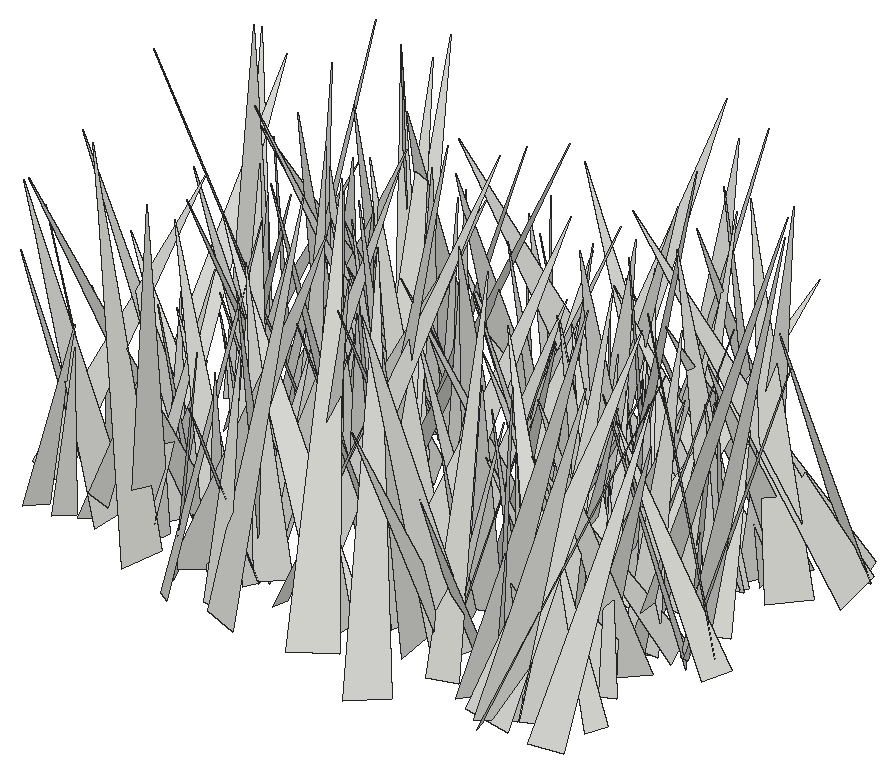
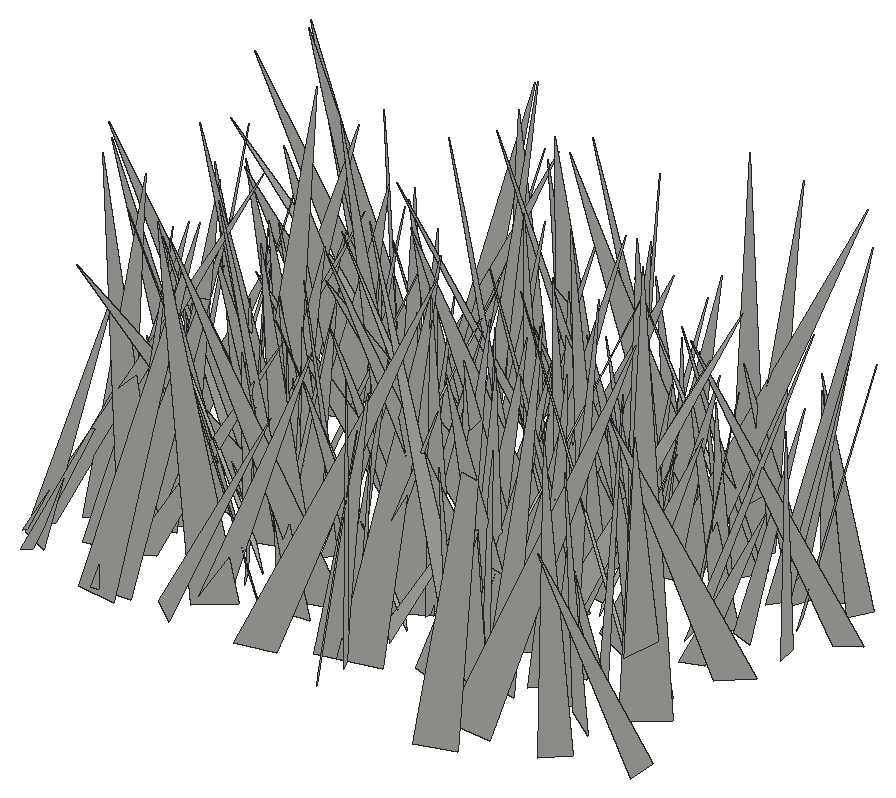
# SketchUp Ruby script. Lengths in inches.
U = 1.inch
M = Sketchup.active_model
def pt(a) = Geom::Point3d.new(a.map { |v| v * U })
def face(e, loops, mat)
  f = e.add_face(loops[0].map { |a| pt(a) })
  loops[1..].each { |l| e.add_face(l.map { |a| pt(a) }).erase! }
  f.material = f.back_material = mat if mat
  f
end
# faces: each face lists its corners as indices into pts; further lists are holes
def faces(e, pts, list, mat = nil) = list.each { |f| face(e, (f[0].is_a?(Array) ? f : [f]).map { |l| l.map { |i| pts[i] } }, mat) }
# xy, xz, yz: faces in a plane at the given z, y or x. An outline is a flat list of corners, or four numbers for a rectangle; further outlines are holes
def ring(l) = l.size == 4 ? [[l[0], l[1]], [l[2], l[1]], [l[2], l[3]], [l[0], l[3]]] : l.each_slice(2).to_a
def flat(e, list, mat, &to3) = list.each { |f| face(e, (f[0].is_a?(Array) ? f : [f]).map { |l| ring(l).map { |u, v| to3.(u, v) } }, mat) }
def xy(e, z, list, mat = nil) = flat(e, list, mat) { |x, y| [x, y, z] }
def xz(e, y, list, mat = nil) = flat(e, list, mat) { |x, z| [x, y, z] }
def yz(e, x, list, mat = nil) = flat(e, list, mat) { |y, z| [x, y, z] }
def lines(e, pts, list) = list.each { |a, b| e.add_line(pt(pts[a]), pt(pts[b])) }
# prism: a flat outline (further loops are holes) pulled along v
def prism(e, loops, v, mat = nil)
  f = face(e, loops, mat); d = Geom::Vector3d.new(v.map { |x| x * U })
  f.pushpull(f.normal.samedirection?(d) ? d.length : -d.length)
end
def box(e, o, s, mat = nil) = prism(e, [[o, [o[0] + s[0], o[1], o[2]], [o[0] + s[0], o[1] + s[1], o[2]], [o[0], o[1] + s[1], o[2]]]], [0, 0, s[2]], mat)
def at(x, y, z, deg = 0) = Geom::Transformation.translation(pt([x, y, z])) * Geom::Transformation.rotation(ORIGIN, Z_AXIS, deg.degrees)
def axes(o, x, y, z) = Geom::Transformation.new([*x, 0, *y, 0, *z, 0, *pt(o).to_a, 1])
def part(name) = M.definitions.add(name)
# library, detail: a bought-in or finely detailed component or shape, given as its bounding box
def library(name, o, s) = part(name).tap { |d| box(d.entities, o, s) }
def detail(e, o, s) = box(e.add_group.entities, o, s)
def put(e, d, t, mat = nil) = e.add_instance(d, t).tap { |i| i.material = mat if mat }
def group(e, t, mat = nil) = e.add_group.tap { |g| g.transformation = t; g.material = mat if mat }.entities
root = M.entities
c1 = part("fur_instance\#9")
p = [[0.8125,0,1.79],[0.67,-0.02,1.48],[0,-0.11,0],[0,0.11,0]]
faces(c1.entities,p,[[0,1,2,3]])
put(root,c1,axes([133.36,44.375,-27.1],[5.70203,-3.94241,1.833],[-4.2894,-5.59456,1.31056],[-0.70959,2.13867,6.80721]))
put(root,c1,axes([129.09,42.8,-27.1],[5.10712,-2.96498,5.20518],[-4.57955,-6.3419,0.88079],[-3.86171,3.59957,5.83935]))
put(root,c1,axes([129.23,47.32,-27.1],[-5.21619,-2.22313,1.39253],[-1.54183,5.10575,2.37575],[2.12232,-1.75473,5.14847]))
put(root,c1,axes([121.18,44.56,-27.1],[0.37459,4.6587,1.44665],[4.87681,-0.39143,-0.00226],[-0.11359,-1.44218,4.67373]))
put(root,c1,axes([120.75,47.14,-27.1],[-2.24525,-3.81491,0.32062],[-3.67914,2.25292,1.04201],[1.05843,-0.26136,4.3022]))
put(root,c1,axes([116.68,46.61,-27.1],[7.00851,-2.19777,2.01204],[-2.01969,-7.2848,-0.92211],[-2.19075,-0.31499,7.28692]))
put(root,c1,axes([129.54,46.98,-27.1],[4.80769,-4.80499,2.60276],[-4.52111,-5.44469,-1.70033],[-3.0695,0.49361,6.58109]))
put(root,c1,axes([132.78,45.19,-27.1],[3.82157,4.19761,2.25189],[4.45533,-4.17126,0.21447],[-1.68552,-1.50865,5.67259]))
put(root,c1,axes([117.2,45.56,-27.1],[-7.37907,1.498,2.27835],[1.63074,7.6926,0.22378],[2.18531,-0.6822,7.52626]))
put(root,c1,axes([121.88,43.93,-27.1],[2.95959,7.19025,1.54721],[7.29869,-3.07695,0.338],[-0.90704,-1.29822,7.76818]))
put(root,c1,axes([113.28,46.3125,-27.1],[2.68413,-2.59886,0.79499],[-2.66781,-2.73276,0.07385],[-0.51851,0.60713,3.7354]))
put(root,c1,axes([112.07,46.29,-27.1],[3.6262,-2.26105,0.60128],[-2.31235,-3.63241,0.28605],[-0.35624,0.56255,4.26378]))
put(root,c1,axes([131.46,46.48,-27.1],[-4.03956,-5.75099,0.92293],[-5.66396,3.6166,-2.25467],[-1.3584,2.0224,6.65646]))
put(root,c1,axes([114.64,47.21,-27.1],[-6.49711,1.14641,2.18071],[1.63194,6.61021,1.38712],[1.84567,-1.80917,6.45001]))
put(root,c1,axes([118.75,45.45,-27.1],[-3.28983,-1.54802,1.9149],[-2.00034,3.5437,-0.57187],[1.43591,1.38997,3.59058]))
put(root,c1,axes([118.43,48.22,-27.1],[-1.35129,-7.71927,0.81651],[-7.46816,1.06686,-2.27338],[-2.11671,1.16382,7.49966]))
put(root,c1,axes([125.51,46.11,-27.1],[-3.60239,-0.15597,0.87969],[-0.19043,3.7046,-0.12301],[0.87288,0.16452,3.60367]))
put(root,c1,axes([136.4,45.98,-27.1],[-3.21224,1.96871,0.46482],[2.01704,3.18335,0.45637],[0.15311,-0.63315,3.7398]))
put(root,c1,axes([120.625,48.03,-27.1],[5.99792,1.55177,2.60045],[2.40829,-5.94226,-2.00876],[-1.83589,-2.72525,5.86071]))
put(root,c1,axes([131.79,45.29,-27.1],[7.44072,-1.6859,2.03296],[-2.09272,-7.4711,1.46382],[-1.61112,1.91833,7.48758]))
put(root,c1,axes([133.125,44.2,-27.1],[-0.55252,7.61083,1.2014],[7.43516,0.84266,-1.91879],[2.02152,-1.01911,7.38568]))
put(root,c1,axes([134.1875,45.31,-27.1],[-5.16392,-1.1559,0.80889],[-1.35151,4.93357,-1.57791],[0.40477,1.72635,5.05098]))
put(root,c1,axes([125.68,44.16,-27.1],[-5.56313,6.05819,1.00831],[6.02083,5.64819,-0.71719],[1.2116,-0.25113,8.19364]))
put(root,c1,axes([114.08,46.72,-27.1],[3.45367,-2.54495,0.42724],[-2.57712,-3.36456,0.79082],[0.1334,0.88889,4.21654]))
put(root,c1,axes([123.74,46.6,-27.1],[6.28963,-0.96384,2.1084],[-1.07131,-6.61487,0.17192],[-2.05588,0.49827,6.36073]))
put(root,c1,axes([118.91,46.125,-27.1],[6.76451,-3.26106,1.25254],[-3.47694,-6.54929,1.72622],[-0.33809,2.1058,7.30844]))
put(root,c1,axes([128.125,46.54,-27.1],[-7.87878,-1.52664,2.20407],[-1.70967,8.13085,-0.47967],[2.06533,0.90687,8.01097]))
put(root,c1,axes([133.12,43.85,-27.1],[6.18332,3.30926,0.01495],[3.17233,-5.93637,1.96995],[-0.9422,1.73008,6.73082]))
put(root,c1,axes([122.71,46.11,-27.1],[3.9235,0.14114,0.37721],[0.06723,-3.8717,0.74932],[-0.3971,0.73898,3.85386]))
put(root,c1,axes([119.34,44.06,-27.1],[4.35483,5.04158,0.80125],[4.65214,-4.35304,2.10539],[-2.1017,0.81089,6.32055]))
put(root,c1,axes([118.79,47.67,-27.1],[3.85883,-1.0172,1.02296],[-0.87371,-3.97244,-0.65425],[-1.14794,-0.39587,3.93665]))
put(root,c1,axes([135.86,43.94,-27.1],[-4.59878,4.14257,0.47856],[3.69105,4.37512,-2.40275],[1.94062,1.49539,5.70408]))
put(root,c1,axes([113.28,48.04,-27.1],[-4.38014,-2.49103,0.91186],[-2.44951,4.47381,0.4553],[1.01814,0.04674,5.01832]))
put(root,c1,axes([129.71,45.99,-27.1],[2.50571,3.8301,0.73521],[3.84486,-2.57244,0.29737],[-0.65369,-0.44905,4.56726]))
put(root,c1,axes([121.5625,47.18,-27.1],[-3.51075,4.42455,2.16586],[4.8357,3.60279,0.47842],[0.94002,-2.00904,5.62789]))
put(root,c1,axes([119.84,46.85,-27.1],[-3.34146,5.15286,1.47209],[5.35695,3.16362,1.08579],[-0.14849,-1.82317,6.0447]))
put(root,c1,axes([116.61,46.14,-27.1],[2.03381,4.83721,0.83738],[4.90479,-2.04045,-0.1258],[-0.20703,-0.82108,5.24587]))
put(root,c1,axes([121.15,46.52,-27.1],[-4.31173,0.11749,0.33288],[0.02447,4.16916,-1.1546],[0.35215,1.14887,4.15592]))
put(root,c1,axes([114.28,47.7,-27.1],[-4.01169,-3.78695,1.3287],[-4.00574,3.89344,-0.9976],[0.2459,1.64323,5.42581]))
put(root,c1,axes([125.25,49.15,-27.1],[-2.82637,-5.01502,0.69558],[-5.06125,2.81969,-0.23605],[0.13409,0.7222,5.75179]))
put(root,c1,axes([132.3,47.21,-27.1],[-3.8319,-0.08961,1.0116],[-0.27638,3.8917,-0.7022],[0.97723,0.7493,3.76807]))
put(root,c1,axes([134.18,46.65,-27.1],[-3.78417,5.30239,0.2634],[5.25954,3.70033,1.07214],[-0.72248,-0.83479,6.42541]))
put(root,c1,axes([124.35,47.18,-27.1],[-4.44973,5.42889,0.1833],[5.21151,4.19987,2.12315],[-1.53186,-1.48148,6.69068]))
put(root,c1,axes([135.0625,49.65,-27.1],[2.07945,-5.56592,1.40736],[-5.43571,-2.39045,-1.42237],[-1.84751,0.76846,5.76892]))
put(root,c1,axes([130.25,45.4,-27.1],[0.51601,7.02264,0.2402],[6.84431,-0.55684,1.57697],[-1.5908,-0.11784,6.86272]))
put(root,c1,axes([120.35,47.71,-27.1],[0.83525,-3.69964,2.10924],[-4.22949,-0.46947,0.8514],[0.49764,2.21949,3.69595]))
put(root,c1,axes([118.83,48.43,-27.1],[-2.76713,3.18046,1.2921],[3.43249,2.58898,0.97827],[0.05304,-1.61979,4.10065]))
put(root,c1,axes([134.68,45.1,-27.1],[-6.77077,3.15469,0.89527],[2.64884,6.47215,-2.77341],[1.93319,2.18084,6.93567]))
put(root,c1,axes([117.28,48.49,-27.1],[-3.57369,-1.9669,1.0397],[-2.0892,3.64317,-0.28897],[0.76478,0.76131,4.06896]))
put(root,c1,axes([128.33,49.34,-27.1],[-3.2792,-1.26365,1.37089],[-0.97388,3.52607,0.9207],[1.58988,-0.44645,3.3915]))
put(root,c1,axes([128.36,50.05,-27.1],[2.49567,-4.97649,0.70111],[-5.02561,-2.47346,0.33254],[-0.01412,0.77585,5.55727]))
put(root,c1,axes([120.59,47.63,-27.1],[4.03025,7.20792,1.49357],[7.34455,-3.82368,-1.36555],[0.49235,-1.96292,8.14446]))
put(root,c1,axes([126.84,47.61,-27.1],[-7.00273,-0.39667,0.95685],[-0.59042,6.90153,-1.45992],[0.85107,1.52402,6.86034]))
put(root,c1,axes([116.36,48.35,-27.1],[-3.76859,1.24193,1.36163],[1.17189,4.00702,-0.41131],[1.42236,-0.01087,3.94658]))
put(root,c1,axes([114.88,49.98,-27.1],[1.3305,-3.93215,0.09517],[-3.71952,-1.22514,1.38031],[1.27907,0.52755,3.91494]))
put(root,c1,axes([135.32,47.95,-27.1],[-0.19051,3.61425,0.52762],[3.57644,0.0773,0.76192],[-0.74175,-0.55561,3.53816]))
put(root,c1,axes([132.47,49.71,-27.1],[-4.25232,-1.15186,0.17503],[-1.13335,4.24309,0.38907],[0.27009,-0.33025,4.38835]))
put(root,c1,axes([114.16,50.06,-27.1],[-1.28236,-4.10189,0.60594],[-4.14572,1.27987,-0.10961],[0.07509,0.61118,4.29626]))
put(root,c1,axes([133.57,49.42,-27.1],[4.86131,-2.02952,0.59697],[-2.06386,-4.87843,0.22145],[-0.46454,0.43544,5.26329]))
put(root,c1,axes([119.67,48.23,-27.1],[-2.53684,6.34204,1.9532],[6.60869,2.60398,0.12835],[0.60133,-1.86275,6.82939]))
put(root,c1,axes([120.46,48.42,-27.1],[3.86814,-0.78573,1.02615],[-1.07279,-3.75781,1.16655],[-0.72076,1.37634,3.77081]))
put(root,c1,axes([135.16,51.9,-27.1],[-5.02387,-1.18033,0.42976],[-0.88594,4.58548,2.23734],[0.8905,-2.09699,4.65046]))
put(root,c1,axes([128.69,47.91,-27.1],[4.75922,3.00167,0.77273],[2.8511,-4.79497,1.06623],[-1.21588,0.50555,5.5248]))
put(root,c1,axes([128.02,50.96,-27.1],[6.9866,-0.46387,0.39437],[-0.38095,-6.874,-1.33651],[-0.47495,-1.31005,6.87325]))
put(root,c1,axes([111.05,48.22,-27.1],[0.65701,6.39206,0.99008],[6.12037,-0.29236,-2.17392],[2.09278,-1.15171,6.04683]))
put(root,c1,axes([134.65,48.33,-27.1],[-3.96377,3.38106,0.80717],[3.27975,4.04327,-0.83051],[1.15166,0.12228,5.14327]))
put(root,c1,axes([120.79,51.24,-27.1],[2.81621,-4.35059,0.38195],[-4.36621,-2.81499,0.12899],[-0.09891,0.39082,5.18093]))
put(root,c1,axes([112.28,49.99,-27.1],[3.8396,0.83392,1.68617],[0.96833,-4.16197,-0.14664],[-1.61273,-0.51356,3.92638]))
put(root,c1,axes([123.21,50.32,-27.1],[-3.81075,-5.76969,1.72606],[-6.01138,3.52106,-1.50194],[-0.36316,2.25903,6.74947]))
put(root,c1,axes([115.74,50.62,-27.1],[-6.60705,-1.5953,0.55499],[-1.61141,6.62494,-0.14037],[0.50631,0.26714,6.79547]))
put(root,c1,axes([135.77,51.5625,-27.1],[-4.16981,-3.31895,0.85743],[-3.36405,4.22145,-0.01946],[0.65859,0.54939,5.32938]))
put(root,c1,axes([122.56,47.89,-27.1],[3.274,7.7332,0.0389],[7.72076,-3.26624,-0.49451],[0.44025,-0.22856,8.38313]))
put(root,c1,axes([130.0625,49.15,-27.1],[4.92859,0.75105,0.39032],[0.57555,-4.66461,1.7081],[-0.62062,1.63853,4.68375]))
put(root,c1,axes([130.85,51.4,-27.1],[4.88822,-0.89007,0.63341],[-0.87396,-4.92864,-0.18113],[-0.65546,-0.06625,4.96529]))
put(root,c1,axes([137.24,51.39,-27.1],[-3.88127,2.88585,0.74535],[2.95869,3.58243,1.53633],[-0.36036,-1.66913,4.58608]))
put(root,c1,axes([117.11,51.57,-27.1],[-3.35519,-0.75879,1.11745],[-0.66434,3.53232,0.40387],[1.17606,-0.1694,3.41613]))
put(root,c1,axes([122.875,50.66,-27.1],[4.94057,6.27292,2.28459],[6.62263,-4.9638,-0.69253],[-0.84236,-2.23369,7.95482]))
put(root,c1,axes([121.28,52.21,-27.1],[4.3252,-1.84495,1.08949],[-1.74272,-4.45705,-0.62914],[-1.2465,-0.1704,4.65998]))
put(root,c1,axes([119.76,50.96,-27.1],[-1.17344,-6.36654,3.3674],[-7.15717,1.41187,0.17527],[0.80444,3.27459,6.4714]))
put(root,c1,axes([133.66,50.3125,-27.1],[-3.54308,4.52564,0.44169],[4.5332,3.47169,0.79207],[-0.35583,-0.83417,5.69276]))
put(root,c1,axes([119.19,51.3,-27.1],[-3.56795,-1.90054,0.20659],[-1.88749,3.43261,-1.0196],[-0.30353,0.99505,3.91187]))
put(root,c1,axes([121.06,52.23,-27.1],[3.12862,-2.29976,0.97047],[-2.27,-3.26853,-0.42753],[-1.03819,0.21622,3.85932]))
put(root,c1,axes([119.6,52.41,-27.1],[-2.97,-5.19915,0.68344],[-5.09037,2.66981,-1.8109],[-1.25951,1.46972,5.70725]))
put(root,c1,axes([134.15,51.15,-27.1],[-0.55684,5.82392,2.02647],[6.12632,0.75415,-0.48394],[0.70204,-1.96161,5.83043]))
put(root,c1,axes([126.51,51.98,-27.1],[-4.66446,-0.17714,0.77084],[-0.14932,4.72517,0.1823],[0.77671,-0.15541,4.66426]))
put(root,c1,axes([135.9,52.88,-27.1],[4.20893,3.73459,3.7879],[4.59902,-4.98198,-0.19834],[-2.67289,-2.69131,5.62342]))
put(root,c1,axes([131.53,53.96,-27.1],[4.41778,-6.32124,1.65754],[-6.32459,-4.6393,-0.83587],[-1.6447,0.86086,7.66656]))
put(root,c1,axes([124.6,53.02,-27.1],[3.18493,-3.37138,0.77047],[-3.44968,-3.17103,0.3845],[-0.24394,0.82581,4.62191]))
put(root,c1,axes([132.14,50.95,-27.1],[-4.57761,1.25738,1.06742],[0.91701,4.55759,-1.43608],[1.37093,1.14988,4.52473]))
put(root,c1,axes([131.1,52.25,-27.1],[1.65832,3.59632,1.35209],[3.82471,-1.68517,-0.20869],[-0.36513,-1.31848,3.95475]))
put(root,c1,axes([125.84,48.96,-27.1],[-5.17652,4.83446,1.05401],[3.91261,4.93311,-3.41105],[3.02894,1.88989,6.20751]))
put(root,c1,axes([114.41,52.42,-27.1],[-3.16167,2.60611,0.16715],[2.5519,3.02748,1.0668],[-0.55458,-0.92652,3.956]))
put(root,c1,axes([118.93,54.9,-27.1],[7.2919,-1.58164,0.56037],[-1.39543,-7.10365,-1.89164],[-0.93186,-1.73896,7.21769]))
put(root,c1,axes([129.96,52.73,-27.1],[-5.05494,-2.22544,0.30278],[-2.23904,4.935,-1.10864],[-0.17591,1.1357,5.41072]))
put(root,c1,axes([127.45,54.4,-27.1],[-5.15654,-2.89646,0.02201],[-2.88562,5.14083,0.47427],[0.2514,-0.40276,5.89529]))
put(root,c1,axes([131.22,51.65,-27.1],[-1.86481,4.13252,0.34952],[4.14724,1.85655,0.17621],[-0.01744,-0.39104,4.53037]))
put(root,c1,axes([130.72,53.49,-27.1],[4.45339,-2.56263,0.11815],[-2.55046,-4.39735,0.75645],[0.27609,0.71411,5.08208]))
put(root,c1,axes([119.44,53.35,-27.1],[-6.03257,-5.76703,0.56772],[-5.59645,5.58532,-2.7307],[-1.50355,2.34912,7.8863]))
put(root,c1,axes([128.52,54.34,-27.1],[-4.47409,-0.55232,0.95951],[-0.288,4.43762,1.21151],[1.069,-1.11608,4.34221]))
put(root,c1,axes([119.45,52.84,-27.1],[5.54301,-4.89223,1.08245],[-4.92161,-5.01325,2.54471],[0.93987,2.60075,6.94141]))
put(root,c1,axes([132.03,54.4,-27.1],[-2.90046,-3.39812,1.38689],[-3.27993,3.19309,0.96417],[1.64705,0.37459,4.36237]))
put(root,c1,axes([133.33,52.5,-27.1],[-4.45117,0.87592,1.04433],[0.68712,4.52233,-0.86441],[1.17717,0.67238,4.45342]))
put(root,c1,axes([117.28,53.11,-27.1],[-0.49335,5.1966,1.87912],[5.02115,-0.36617,2.33091],[-2.30734,-1.90798,4.67065]))
put(root,c1,axes([134.33,50.77,-27.1],[7.79418,1.63756,2.08164],[0.8535,-7.67768,2.8441],[-2.50726,2.47704,7.43922]))
put(root,c1,axes([123.875,55.66,-27.1],[4.30968,-5.09044,0.61484],[-5.06109,-4.35201,-0.55619],[-0.82219,0.10671,6.64655]))
put(root,c1,axes([113.53,55.09,-27.1],[6.27835,0.76334,0.54412],[0.88551,-6.03847,-1.74618],[-0.30762,-1.80294,6.07875]))
put(root,c1,axes([116.91,55.76,-27.1],[-0.2881,-6.79413,1.19024],[-6.52945,0.65262,2.14482],[2.22333,1.03623,6.45314]))
put(root,c1,axes([130.15,54.78,-27.1],[-3.55733,-3.55392,1.20149],[-3.66341,3.64755,-0.05732],[0.80828,0.89081,5.02808]))
put(root,c1,axes([114.26,55.1,-27.1],[1.4923,-4.43759,0.64343],[-4.35505,-1.27294,1.3215],[1.06759,1.01025,4.49142]))
put(root,c1,axes([118.21,53.71,-27.1],[3.92442,2.27765,0.90763],[2.32456,-4.0011,-0.01041],[-0.77966,-0.46478,4.53747]))
put(root,c1,axes([129.31,54.79,-27.1],[1.81609,-4.28388,1.69446],[-4.45246,-2.09973,-0.53642],[-1.18256,1.32684,4.62191]))
put(root,c1,axes([135.65,52.18,-27.1],[-6.79191,0.51616,3.38033],[-0.49773,7.28774,-2.11287],[3.3831,2.10844,6.47551]))
put(root,c1,axes([131.38,52.75,-27.1],[7.46967,2.68884,2.29218],[2.3982,-7.79505,1.32883],[-2.59473,0.53597,7.82688]))
put(root,c1,axes([124.96,53.71,-27.1],[0.90877,4.85728,1.17196],[4.86719,-0.59112,-1.32422],[1.13009,-1.36012,4.76083]))
put(root,c1,axes([122.35,53.99,-27.1],[-5.92125,2.00992,1.02968],[2.02644,6.00419,-0.06686],[0.99676,-0.26678,6.25272]))
put(root,c1,axes([135.64,53.51,-27.1],[-2.23531,2.8422,0.49749],[2.78374,2.28983,-0.57415],[0.75919,-0.0278,3.57002]))
put(root,c1,axes([135.74,51.625,-27.1],[4.27823,3.00126,0.70858],[2.21616,-3.83495,2.86263],[-2.14435,2.02448,4.3722]))
put(root,c1,axes([131.73,54.07,-27.1],[5.13146,2.31605,0.71954],[2.33013,-5.17519,0.0403],[-0.67253,-0.25897,5.62978]))
put(root,c1,axes([121.19,56.51,-27.1],[-6.73685,-3.71008,0.0403],[-3.70619,6.73292,0.28887],[0.17463,-0.23362,7.68547]))
put(root,c1,axes([123.37,54.78,-27.1],[5.69837,-0.41307,2.53776],[-0.52377,-6.22748,0.16244],[-2.51724,0.36068,5.71101]))
put(root,c1,axes([133.03,55.47,-27.1],[4.02483,1.17033,1.17041],[1.40502,-4.04247,-0.78939],[-0.87491,-1.10794,4.11653]))
put(root,c1,axes([134.375,55.41,-27.1],[-3.74193,-1.93414,1.83822],[-1.95383,4.14237,0.38123],[1.81727,0.47108,4.19495]))
put(root,c1,axes([131.4,54.95,-27.1],[1.02394,3.35387,1.44831],[3.57422,-1.23084,0.32333],[-0.75567,-1.27715,3.49176]))
put(root,c1,axes([112.5625,52.39,-27.1],[-2.48989,6.58556,0.19317],[6.42005,2.47161,-1.51018],[1.47984,0.3578,6.87667]))
put(root,c1,axes([113.17,56.46,-27.1],[4.71718,-6.41333,2.08506],[-6.64537,-4.85367,0.10513],[-1.14777,1.74389,7.96063]))
put(root,c1,axes([113.81,56.14,-27.1],[4.65785,-0.69082,1.21899],[-0.53967,-4.78978,-0.65231],[-1.29303,-0.48941,4.6634]))
put(root,c1,axes([133.98,56.05,-27.1],[4.51203,-4.20905,2.90182],[-4.30887,-5.21386,-0.8628],[-2.75143,1.26279,6.10984]))
put(root,c1,axes([119.36,56.32,-27.1],[-4.57691,0.82768,1.57562],[1.18388,4.66198,0.99001],[1.32893,-1.30255,4.54457]))
put(root,c1,axes([115.57,55.76,-27.1],[-3.42106,-4.15596,2.05732],[-4.44833,3.66341,0.00339],[1.31032,1.58608,5.3829]))
put(root,c1,axes([133.96,56.33,-27.1],[0.76269,-3.95415,0.89534],[-4.04548,-0.80213,-0.09639],[-0.26648,0.86018,4.02588]))
put(root,c1,axes([114.61,56.68,-27.1],[5.46808,5.3055,1.78388],[5.41419,-4.38056,-3.56761],[1.42026,-3.72732,6.73205]))
put(root,c1,axes([116.31,53.5,-27.1],[-5.10797,-4.03263,5.02727],[-5.71036,5.80586,-1.14484],[2.98787,4.202,6.40647]))
put(root,c1,axes([126.93,55.35,-27.1],[3.29579,4.51514,1.8086],[4.80118,-3.36974,-0.33663],[-0.7786,-1.66678,5.57991]))
put(root,c1,axes([115.91,57.625,-27.1],[6.82649,-0.20783,2.36031],[0.47416,-6.93274,-1.9818],[-2.32152,-2.02711,6.5358]))
put(root,c1,axes([129.52,55.02,-27.1],[-4.01098,-1.65554,1.8183],[-2.11594,4.09606,-0.93811],[1.25294,1.61753,4.23659]))
put(root,c1,axes([117.26,56.7,-27.1],[4.37094,-3.26497,1.75227],[-3.26747,-4.6741,-0.55863],[-1.74761,0.57306,5.42707]))
put(root,c1,axes([119.2,58.2,-27.1],[1.9027,-5.40071,0.1352],[-5.35593,-1.9045,-0.70218],[-0.70705,-0.10684,5.68285]))
put(root,c1,axes([134.92,58.55,-27.1],[3.41213,-4.67618,0.33772],[-4.46229,-3.36731,-1.54031],[-1.43828,-0.64649,5.58003]))
put(root,c1,axes([129.73,57.22,-27.1],[4.8829,2.83209,2.83107],[3.60518,-5.05239,-1.16384],[-1.7431,-2.51617,5.52349]))
put(root,c1,axes([119.6,58.67,-27.1],[-3.6044,-3.37024,0.34721],[-3.01204,3.4196,1.92476],[1.55135,-1.19103,4.54373]))
put(root,c1,axes([120.65,55.15,-27.1],[7.61599,0.93725,0.32253],[0.89381,-7.57423,0.90437],[-0.42844,0.85927,7.61996]))
put(root,c1,axes([131.21,53.43,-27.1],[-1.51427,6.54379,0.36236],[5.84338,1.51647,-2.96661],[2.96773,0.35306,6.02606]))
put(root,c1,axes([133.4,53.97,-27.1],[1.19903,6.87384,0.5978],[6.78552,-1.2847,1.16229],[-1.25048,-0.38022,6.88014]))
put(root,c1,axes([121.6,53.28,-27.1],[-6.67493,4.02137,0.12146],[3.83511,6.43107,-2.16198],[1.21576,1.79188,7.48679]))
put(root,c1,axes([127.54,57.16,-27.1],[3.13574,-5.33007,1.5739],[-5.55752,-3.01682,0.85589],[-0.02918,1.79133,6.12454]))
put(root,c1,axes([118.34,57.85,-27.1],[-1.31696,-6.51866,1.83434],[-6.75362,1.40125,0.13086],[0.49623,1.77078,6.64907]))
put(root,c1,axes([137.375,58.78,-27.1],[-8.16776,0.06376,0.0825],[0.08376,7.86119,2.21763],[0.06209,-2.2183,7.8612]))
put(root,c1,axes([130.9,55.06,-27.1],[-2.1836,4.82414,0.14178],[4.82373,2.17653,0.23433],[-0.15514,-0.2257,5.29014]))
put(root,c1,axes([123.6875,57.15,-27.1],[-2.7685,-2.84273,0.0732],[-2.6967,2.59213,-1.32656],[-0.90237,0.97511,3.73978]))
put(root,c1,axes([123.1,59.41,-27.1],[2.89826,-6.60565,0.55734],[-6.55377,-2.94663,-0.84295],[-0.99662,0.16719,7.16407]))
put(root,c1,axes([125.18,57.51,-27.1],[4.42222,0.57042,2.59632],[0.96066,-5.04183,-0.52855],[-2.47858,-0.93641,4.42741]))
put(root,c1,axes([119.11,58.63,-27.1],[8.07507,1.50255,0.4439],[1.56674,-7.73574,-2.31627],[0.00564,-2.35841,7.88031]))
put(root,c1,axes([123.63,56.29,-27.1],[4.56915,3.9518,0.34933],[3.96081,-4.51383,-0.74378],[0.22516,-0.79028,5.99505]))
put(root,c1,axes([135.98,56.88,-27.1],[-4.89648,5.17695,2.06152],[5.4889,4.95404,0.59637],[0.96057,-1.91907,7.10075]))
put(root,c1,axes([125.12,56.01,-27.1],[-0.69382,4.82103,0.91338],[4.82167,0.84094,-0.77604],[0.90996,-0.78004,4.80848]))
put(root,c1,axes([114.05,55.48,-27.1],[-5.08982,4.44528,0.70369],[4.40622,5.13821,-0.58816],[0.91699,-0.01575,6.73207]))
put(root,c1,axes([132.63,60.85,-27.1],[4.86562,-4.5964,0.06859],[-4.19123,-4.47675,-2.68294],[-1.88818,-1.90726,6.13213]))
put(root,c1,axes([124.48,58.08,-27.1],[-4.64353,0.24048,0.81476],[0.40253,4.60984,0.93348],[0.74809,-0.98772,4.55508]))
put(root,c1,axes([117.37,60.73,-27.1],[2.70234,-6.75975,0.1599],[-6.39067,-2.60962,-2.31767],[-2.20886,-0.71979,6.90111]))
put(root,c1,axes([121.1875,55.0625,-27.1],[-7.30125,2.0292,0.54339],[1.84392,7.1322,-1.85816],[1.00641,1.65384,7.34664]))
put(root,c1,axes([126.63,58.19,-27.1],[3.82304,5.79974,2.60132],[6.29108,-3.01834,-2.51622],[0.9089,-3.50316,6.47466]))
put(root,c1,axes([133.48,58.16,-27.1],[-5.14523,1.96025,0.06602],[1.88898,4.90265,1.64806],[-0.52792,-1.56261,5.25356]))
put(root,c1,axes([134.15,57.43,-27.1],[6.73151,-1.98165,2.55494],[-2.23492,-7.11595,0.36912],[-2.33662,1.09735,7.00742]))
put(root,c1,axes([119.16,58.31,-27.1],[5.28351,-1.61661,1.62366],[-1.56193,-5.52709,-0.42043],[-1.67632,0.05465,5.50927]))
put(root,c1,axes([120.97,58.59,-27.1],[-0.75955,-3.70224,0.74684],[-3.72635,0.61048,-0.76351],[-0.61539,0.87293,3.70143]))
put(root,c1,axes([125.07,56.875,-27.1],[-3.90269,-1.36809,1.23152],[-1.73858,3.68797,-1.41263],[0.60468,1.77384,3.88679]))
put(root,c1,axes([119.1,57.67,-27.1],[4.24793,5.0228,3.04998],[5.34423,-4.86703,0.57187],[-2.44337,-1.91294,6.55335]))
put(root,c1,axes([120.46,55.02,-27.1],[-0.64935,7.68845,0.01437],[7.6155,0.6412,1.06165],[-1.05669,-0.10353,7.64243]))
put(root,c1,axes([134.51,57.61,-27.1],[-6.69372,-1.63538,1.73187],[-1.91789,6.76382,-1.02573],[1.41263,1.43387,6.81383]))
put(root,c1,axes([126.54,60.72,-27.1],[-6.66712,2.68909,2.42043],[3.53397,5.92752,3.14894],[0.77508,-3.89533,6.46266]))
put(root,c1,axes([130.28,55.83,-27.1],[5.47327,5.90798,0.9862],[5.7796,-5.55993,1.23167],[-1.57262,0.12835,7.95889]))
put(root,c1,axes([128.42,58.23,-27.1],[4.16572,3.95636,0.93283],[4.06431,-4.03236,-1.04767],[0.06588,-1.40123,5.64875]))
put(root,c1,axes([136.89,59.65,-27.1],[-1.73362,-4.79917,0.85478],[-4.86621,1.65027,-0.60395],[-0.28757,1.00633,5.06683]))
put(root,c1,axes([120.16,58.07,-27.1],[1.76175,3.91399,1.38102],[4.01071,-1.99148,0.5277],[-1.06803,-1.02224,4.25965]))
put(root,c1,axes([136.75,60.26,-27.1],[-3.56897,-0.50146,0.42511],[-0.28446,3.29362,1.49696],[0.59267,-1.43888,3.27843]))
put(root,c1,axes([113.99,60.28,-27.1],[4.00821,-3.73033,0.31245],[-3.73197,-4.01777,-0.09299],[-0.29215,0.14465,5.47471]))
put(root,c1,axes([124.15,59.6875,-27.1],[1.70929,-4.46495,1.67991],[-4.63149,-1.98085,-0.55231],[-1.1433,1.34907,4.74893]))
put(root,c1,axes([132.97,61.21,-27.1],[-0.03159,-6.8611,0.78211],[-6.88005,-0.03586,-0.59249],[-0.59273,0.78192,6.83555]))
put(root,c1,axes([114.78,57.98,-27.1],[2.34142,5.16985,1.64131],[5.10687,-2.70355,1.23051],[-1.82787,-0.93109,5.54034]))
put(root,c1,axes([126.36,57.04,-27.1],[0.38295,8.08113,1.09098],[7.9956,-0.1576,-1.6392],[1.60161,-1.14545,7.92239]))
put(root,c1,axes([123.53,59.55,-27.1],[-4.21315,-2.34987,2.26772],[-2.4638,4.71684,0.31027],[2.14339,0.80291,4.81418]))
put(root,c1,axes([129.85,58.8,-27.1],[-6.207,1.9177,0.03314],[1.91765,6.20287,0.22937],[-0.03607,-0.22893,6.49244]))
put(root,c1,axes([117.54,62.3125,-27.1],[2.10072,-7.09935,0.00934],[-7.09522,-2.09917,0.25546],[0.24231,0.08144,7.39923]))
put(root,c1,axes([129.44,59.25,-27.1],[3.63637,-5.76719,3.12725],[-6.51934,-3.57646,0.98508],[-0.73369,3.19558,6.74635]))
put(root,c1,axes([111.13,59.21,-27.1],[4.26787,-0.90452,0.30078],[-0.95208,-4.11231,1.14272],[-0.04649,1.18073,4.21035]))
put(root,c1,axes([130.48,60.72,-27.1],[-2.43952,-3.83837,0.4143],[-3.75379,2.24378,-1.31547],[-0.90209,1.04325,4.3536]))
put(root,c1,axes([123.49,61.21,-27.1],[-3.34648,-2.86729,1.25208],[-2.75468,3.56945,0.81158],[1.4835,0.16004,4.33146]))
